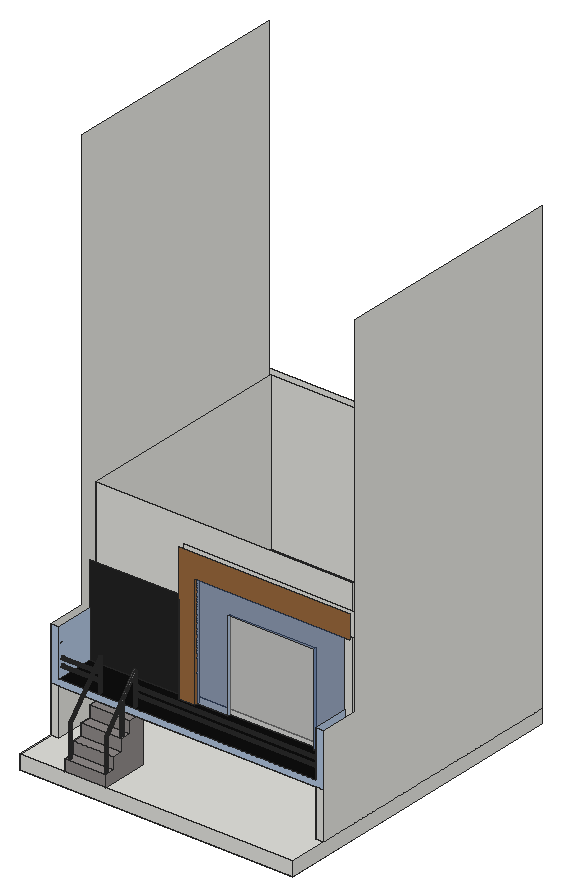
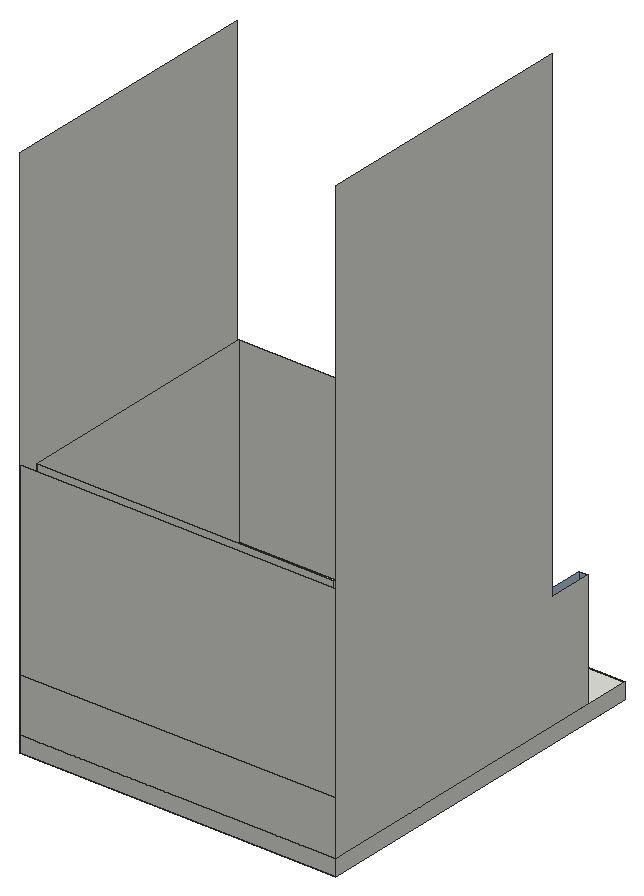
# SketchUp Ruby script. Lengths in inches.
U = 1.inch
M = Sketchup.active_model
def pt(a) = Geom::Point3d.new(a.map { |v| v * U })
def face(e, loops, mat)
  f = e.add_face(loops[0].map { |a| pt(a) })
  loops[1..].each { |l| e.add_face(l.map { |a| pt(a) }).erase! }
  f.material = f.back_material = mat if mat
  f
end
# faces: each face lists its corners as indices into pts; further lists are holes
def faces(e, pts, list, mat = nil) = list.each { |f| face(e, (f[0].is_a?(Array) ? f : [f]).map { |l| l.map { |i| pts[i] } }, mat) }
# xy, xz, yz: faces in a plane at the given z, y or x. An outline is a flat list of corners, or four numbers for a rectangle; further outlines are holes
def ring(l) = l.size == 4 ? [[l[0], l[1]], [l[2], l[1]], [l[2], l[3]], [l[0], l[3]]] : l.each_slice(2).to_a
def flat(e, list, mat, &to3) = list.each { |f| face(e, (f[0].is_a?(Array) ? f : [f]).map { |l| ring(l).map { |u, v| to3.(u, v) } }, mat) }
def xy(e, z, list, mat = nil) = flat(e, list, mat) { |x, y| [x, y, z] }
def xz(e, y, list, mat = nil) = flat(e, list, mat) { |x, z| [x, y, z] }
def yz(e, x, list, mat = nil) = flat(e, list, mat) { |y, z| [x, y, z] }
def lines(e, pts, list) = list.each { |a, b| e.add_line(pt(pts[a]), pt(pts[b])) }
# prism: a flat outline (further loops are holes) pulled along v
def prism(e, loops, v, mat = nil)
  f = face(e, loops, mat); d = Geom::Vector3d.new(v.map { |x| x * U })
  f.pushpull(f.normal.samedirection?(d) ? d.length : -d.length)
end
def box(e, o, s, mat = nil) = prism(e, [[o, [o[0] + s[0], o[1], o[2]], [o[0] + s[0], o[1] + s[1], o[2]], [o[0], o[1] + s[1], o[2]]]], [0, 0, s[2]], mat)
def at(x, y, z, deg = 0) = Geom::Transformation.translation(pt([x, y, z])) * Geom::Transformation.rotation(ORIGIN, Z_AXIS, deg.degrees)
def axes(o, x, y, z) = Geom::Transformation.new([*x, 0, *y, 0, *z, 0, *pt(o).to_a, 1])
def part(name) = M.definitions.add(name)
# library, detail: a bought-in or finely detailed component or shape, given as its bounding box
def library(name, o, s) = part(name).tap { |d| box(d.entities, o, s) }
def detail(e, o, s) = box(e.add_group.entities, o, s)
def put(e, d, t, mat = nil) = e.add_instance(d, t).tap { |i| i.material = mat if mat }
def group(e, t, mat = nil) = e.add_group.tap { |g| g.transformation = t; g.material = mat if mat }.entities
root = M.entities
M.materials.add("[0099_LightSteelBlue]").color = [176, 196, 222]
M.materials.add("[0136_Charcoal]").color = [35, 35, 35]
M.materials.add("[Granite Dark Gray]").color = [15, 15, 15]
M.materials.add("[Metal Corrugated Shiny]").color = [124, 124, 124]
M.materials.add("[Stone Marble]").color = [143, 138, 136]
M.materials.add("[Translucent Glass Blue]").color = [59, 88, 140]
M.materials["[Translucent Glass Blue]"].alpha = 0.5
M.materials.add("[Translucent Glass Gray]").color = [173, 173, 173]
M.materials["[Translucent Glass Gray]"].alpha = 0.5
M.materials.add("[Wood Floor]").color = [155, 105, 61]
xy(root,0,[[0,0,420,480]])
xy(root,21,[[0,0,69.34,0,69.34,72,132,72,132,0,420,0,420,60,408,60,408,468,12,468,12,60,0,60],[0,60,0,480,420,480,420,60,408,60,408,468,12,468,12,60]])
xy(root,39,[[73.02,4.13,72.5,4.2,72.02,4.4,71.61,4.71,71.29,5.13,71.09,5.61,71.02,6.13,71.09,6.64,71.29,7.13,71.61,7.54,72.02,7.86,72.5,8.06,73.02,8.13,73.54,8.06,74.02,7.86,74.44,7.54,74.75,7.13,74.95,6.64,75.02,6.13,74.95,5.61,74.75,5.13,74.44,4.71,74.02,4.4,73.54,4.2],[128.75,4.13,128.77,4.13,129,4.16],[128.49,4.16,128.23,4.21,128.25,4.2],[129.26,4.19,129.29,4.2,129.51,4.29],[127.99,4.3,127.75,4.41,127.77,4.4],
  [129.75,4.39,129.77,4.4,129.96,4.54],[127.54,4.57,127.34,4.73,127.36,4.71],[130.17,4.7,130.19,4.71,130.33,4.9],[127.18,4.94,127.03,5.15,127.04,5.13],[130.49,5.11,130.5,5.13,130.59,5.35],
  [126.93,5.39,126.84,5.64,126.84,5.61],[130.69,5.59,130.7,5.61,130.73,5.84],[126.8,5.89,126.77,6.15,126.77,6.13],[130.77,6.1,130.77,6.13,130.74,6.36],[126.81,6.41,126.85,6.67,126.84,6.64],
  [130.71,6.62,130.7,6.64,130.61,6.86],[126.95,6.91,127.05,7.15,127.04,7.13],[130.51,7.1,130.5,7.13,130.36,7.3125],[127.21,7.35,127.38,7.56,127.36,7.54],[130.2,7.52,130.19,7.54,130,7.68],
  [127.58,7.72,127.79,7.87,127.77,7.86],[129.79,7.84,129.77,7.86,129.55,7.95],[128.04,7.97,128.28,8.0625,128.25,8.06],[129.3125,8.05,129.29,8.06,129.06,8.09],[128.54,8.1,128.8,8.125,128.77,8.13]])
xy(root,39,[[[69.34,0,132,16],[128.72,4.13,128.49,4.16,128.25,4.2,128.23,4.21,128.2,4.21,127.99,4.3,127.77,4.4,127.73,4.42,127.54,4.57,127.36,4.71,127.32,4.75,127.04,5.13,127.03,5.15,127.01,5.17,126.93,5.39,126.84,5.61,126.84,5.64,126.83,5.66,126.8,5.89,126.77,6.13,126.77,6.18,126.81,6.41,126.84,6.64,126.85,6.67,126.85,6.69,126.95,6.91,127.04,7.13,127.05,7.15,127.07,7.17,127.21,7.35,127.36,7.54,127.38,7.56,127.39,7.58,127.77,7.86,127.79,7.87,127.82,7.88,128.04,7.97,128.25,8.06,128.28,8.0625,128.3,8.07,128.54,8.1,128.77,8.13,128.8,8.125,128.82,8.125,129.06,8.09,129.29,8.06,129.3125,8.05,129.34,8.05,129.55,7.95,129.77,7.86,129.79,7.84,129.82,7.83,130,7.68,130.19,7.54,130.2,7.52,130.22,7.5,130.36,7.3125,130.5,7.13,130.51,7.1,130.53,7.08,130.61,6.86,130.7,6.64,130.72,6.6,130.74,6.36,130.77,6.13,130.77,6.08,130.73,5.84,130.7,5.61,130.69,5.59,130.6875,5.56,130.59,5.35,130.5,5.13,130.49,5.11,130.48,5.08,130.33,4.9,130.19,4.71,130.17,4.7,130.15,4.68,129.77,4.4,129.75,4.39,129.73,4.37,129.51,4.29,129.29,4.2,129.26,4.19,129.24,4.18,129,4.16,128.77,4.13],[73.02,4.13,72.5,4.2,72.02,4.4,71.61,4.71,71.29,5.13,71.09,5.61,71.02,6.13,71.09,6.64,71.29,7.13,71.61,7.54,72.02,7.86,72.5,8.06,73.02,8.13,73.54,8.06,74.02,7.86,74.44,7.54,74.75,7.13,74.95,6.64,75.02,6.13,74.95,5.61,74.75,5.13,74.44,4.71,74.02,4.4,73.54,4.2]]],"[Stone Marble]")
xy(root,57,[[69.34,16,132,30.4375]],"[Stone Marble]")
xy(root,75,[[127.2,35.08,126.68,35.15,126.2,35.35,125.78,35.67,125.46,36.08,125.26,36.5625,125.2,37.08,125.26,37.6,125.46,38.08,125.78,38.49,126.2,38.8125,126.68,39.01,127.2,39.08,127.71,39.01,128.2,38.8125,128.61,38.49,128.93,38.08,129.13,37.6,129.2,37.08,129.13,36.5625,128.93,36.08,128.61,35.67,128.2,35.35,127.71,35.15]])
xy(root,75,[[[69.34,30.4375,132,47.125],[127.2,35.08,126.68,35.15,126.2,35.35,125.78,35.67,125.46,36.08,125.26,36.5625,125.2,37.08,125.26,37.6,125.46,38.08,125.78,38.49,126.2,38.8125,126.68,39.01,127.2,39.08,127.71,39.01,128.2,38.8125,128.61,38.49,128.93,38.08,129.13,37.6,129.2,37.08,129.13,36.5625,128.93,36.08,128.61,35.67,128.2,35.35,127.71,35.15]]],"[Stone Marble]")
xy(root,93,[[12,60,12,468,408,468,408,60,132,60,132,72,69.34,72,69.34,60],[69.34,60,132,72]])
xy(root,93,[[69.34,47.125,132,60]],"[Stone Marble]")
xy(root,103,[[72.44,62.83,71.92,62.9,71.44,63.1,71.03,63.42,70.71,63.83,70.51,64.32,70.44,64.83,70.51,65.35,70.71,65.83,71.03,66.25,71.44,66.57,71.92,66.77,72.44,66.83,72.96,66.77,73.44,66.57,73.86,66.25,74.17,65.83,74.375,65.35,74.44,64.83,74.375,64.32,74.17,63.83,73.86,63.42,73.44,63.1,72.96,62.9],[126.03,62.85,125.51,62.86,125.01,63.01,124.56,63.28,124.2,63.66,123.95,64.11,123.83,64.62,123.84,65.14,123.99,65.64,124.26,66.09,124.64,66.45,125.1,66.7,125.6,66.82,126.125,66.81,126.625,66.66,127.07,66.39,127.43,66.01,127.68,65.55,127.8,65.05,127.79,64.52,127.64,64.02,127.37,63.58,126.99,63.22,126.54,62.97],[156,111,180,120],[12,132,408,468]])
xy(root,103,[[[12,60,408,60,408,116,360,116,360,120,228,120,228,116,180,116,180,111,156,111,156,120,12,120],[72.44,62.83,71.92,62.9,71.44,63.1,71.03,63.42,70.71,63.83,70.51,64.32,70.44,64.83,70.51,65.35,70.71,65.83,71.03,66.25,71.44,66.57,71.92,66.77,72.44,66.83,72.96,66.77,73.44,66.57,73.86,66.25,74.17,65.83,74.375,65.35,74.44,64.83,74.375,64.32,74.17,63.83,73.86,63.42,73.44,63.1,72.96,62.9],[126.03,62.85,125.51,62.86,125.01,63.01,124.56,63.28,124.2,63.66,123.95,64.11,123.83,64.62,123.84,65.14,123.99,65.64,124.26,66.09,124.64,66.45,125.1,66.7,125.6,66.82,126.125,66.81,126.625,66.66,127.07,66.39,127.43,66.01,127.68,65.55,127.8,65.05,127.79,64.52,127.64,64.02,127.37,63.58,126.99,63.22,126.54,62.97]]],"[Granite Dark Gray]")
xy(root,121.24,[[127.2,35.08,127.71,35.15,128.2,35.35,128.61,35.67,128.93,36.08,129.13,36.5625,129.2,37.08,129.13,37.6,128.93,38.08,128.61,38.49,128.2,38.8125,127.71,39.01,127.2,39.08,126.68,39.01,126.2,38.8125,125.78,38.49,125.46,38.08,125.26,37.6,125.2,37.08,125.26,36.5625,125.46,36.08,125.78,35.67,126.2,35.35,126.68,35.15]])
xz(root,0,[[0,0,420,21]])
xz(root,0,[[69.34,21,132,39]],"[Stone Marble]")
xz(root,16,[[69.34,39,132,57]],"[Stone Marble]")
xz(root,30.4375,[[69.34,57,132,75]],"[Stone Marble]")
xz(root,47.125,[[69.34,75,132,93]],"[Stone Marble]")
xz(root,60,[[0,21,12,93],[408,21,420,93]])
xz(root,60,[[0,93,420,93,420,175,408,175,408,103,12,103,12,175,0,175]],"[0099_LightSteelBlue]")
xz(root,72,[[69.34,21,132,93]])
xz(root,111,[[156,103,180,103,180,277,420,277,420,313,156,313]],"[Wood Floor]")
xz(root,116,[[180,103,228,103,228,241,360,241,360,103,408,103,408,277,180,277]],"[Translucent Glass Blue]")
xz(root,120,[[156,103,156,313,420,313,420,277,180,277,180,103]])
xz(root,120,[[12,103,156,241]],"[0136_Charcoal]")
xz(root,120,[[228,103,360,241]],"[Translucent Glass Gray]")
xz(root,132,[[12,103,408,343]])
xz(root,468,[[12,21,408,93],[12,103,408,343]])
xz(root,480,[[0,0,420,21],[0,21,420,93],[0,93,420,343]])
yz(root,0,[[0,0,480,21],[60,21,60,175,120,175,120,823,480,823,480,21]])
yz(root,12,[[60,21,468,93],[132,103,468,343],[64.83,116.9375,64.32,117.01,63.83,117.21,63.42,117.52,63.1,117.9375,62.9,118.42,62.83,118.9375,62.9,119.46,63.1,119.9375,63.42,120.35,63.83,120.67,64.32,120.87,64.83,120.9375,65.35,120.87,65.83,120.67,66.25,120.35,66.57,119.9375,66.77,119.46,66.83,118.9375,66.77,118.42,66.57,117.9375,66.25,117.52,65.83,117.21,65.35,117.01],[64.83,127.875,64.32,127.94,63.83,128.14,63.42,128.46,63.1,128.875,62.9,129.36,62.83,129.875,62.9,130.39,63.1,130.875,63.42,131.29,63.83,131.61,64.32,131.81,64.83,131.875,65.35,131.81,65.83,131.61,66.25,131.29,66.57,130.875,66.77,130.39,66.83,129.875,66.77,129.36,66.57,128.875,66.25,128.46,65.83,128.14,65.35,127.94]])
yz(root,12,[[[60,103,120,175],[64.83,116.9375,64.32,117.01,63.83,117.21,63.42,117.52,63.1,117.9375,62.9,118.42,62.83,118.9375,62.9,119.46,63.1,119.9375,63.42,120.35,63.83,120.67,64.32,120.87,64.83,120.9375,65.35,120.87,65.83,120.67,66.25,120.35,66.57,119.9375,66.77,119.46,66.83,118.9375,66.77,118.42,66.57,117.9375,66.25,117.52,65.83,117.21,65.35,117.01],[64.83,127.875,64.32,127.94,63.83,128.14,63.42,128.46,63.1,128.875,62.9,129.36,62.83,129.875,62.9,130.39,63.1,130.875,63.42,131.29,63.83,131.61,64.32,131.81,64.83,131.875,65.35,131.81,65.83,131.61,66.25,131.29,66.57,130.875,66.77,130.39,66.83,129.875,66.77,129.36,66.57,128.875,66.25,128.46,65.83,128.14,65.35,127.94],[64.83,138.5625,64.32,138.63,63.83,138.83,63.42,139.15,63.1,139.5625,62.9,140.05,62.83,140.5625,62.9,141.08,63.1,141.5625,63.42,141.98,63.83,142.3,64.32,142.5,64.83,142.5625,65.35,142.5,65.83,142.3,66.25,141.98,66.57,141.5625,66.77,141.08,66.83,140.5625,66.77,140.05,66.57,139.5625,66.25,139.15,65.83,138.83,65.35,138.63],[64.83,149.25,64.32,149.32,63.83,149.52,63.42,149.84,63.1,150.25,62.9,150.73,62.83,151.25,62.9,151.77,63.1,152.25,63.42,152.67,63.83,152.98,64.32,153.18,64.83,153.25,65.35,153.18,65.83,152.98,66.25,152.67,66.57,152.25,66.77,151.77,66.83,151.25,66.77,150.73,66.57,150.25,66.25,149.84,65.83,149.52,65.35,149.32]]],"[0099_LightSteelBlue]")
yz(root,69.34,[[0,21,0,39,16,39,16,57,30.4375,57,30.4375,75,47.125,75,47.125,93,72,93,72,21]],"[Stone Marble]")
yz(root,132,[[0,21,72,21,72,93,47.125,93,47.125,75,30.4375,75,30.4375,57,16,57,16,39,0,39]],"[Stone Marble]")
yz(root,156,[[111,103,120,241]])
yz(root,180,[[116,103,120,277]])
yz(root,180,[[111,103,116,277]],"[Wood Floor]")
yz(root,228,[[116,103,120,241]],"[0099_LightSteelBlue]")
yz(root,360,[[116,103,120,241]],"[0099_LightSteelBlue]")
yz(root,408,[[60,21,468,93],[132,103,468,343],[64.83,117.19,65.29,117.25,65.71,117.42,66.07,117.7,66.35,118.06,66.52,118.49,66.58,118.9375,66.52,119.39,66.35,119.8125,66.07,120.18,65.71,120.45,65.29,120.63,64.83,120.6875,64.38,120.63,63.96,120.45,63.6,120.18,63.32,119.8125,63.14,119.39,63.08,118.9375,63.14,118.49,63.32,118.06,63.6,117.7,63.96,117.42,64.38,117.25],[64.83,127.98,65.32,128.05,65.78,128.24,66.17,128.54,66.47,128.93,66.66,129.39,66.73,129.875,66.66,130.37,66.47,130.82,66.17,131.21,65.78,131.52,65.32,131.7,64.83,131.77,64.34,131.7,63.89,131.52,63.5,131.21,63.2,130.82,63.01,130.37,62.94,129.875,63.01,129.39,63.2,128.93,63.5,128.54,63.89,128.24,64.34,128.05]])
yz(root,408,[[[60,103,116,175],[64.83,138.5625,65.35,138.63,65.83,138.83,66.25,139.15,66.57,139.5625,66.77,140.05,66.83,140.5625,66.77,141.08,66.57,141.5625,66.25,141.98,65.83,142.3,65.35,142.5,64.83,142.5625,64.32,142.5,63.83,142.3,63.42,141.98,63.1,141.5625,62.9,141.08,62.83,140.5625,62.9,140.05,63.1,139.5625,63.42,139.15,63.83,138.83,64.32,138.63],[64.83,149.25,65.35,149.32,65.83,149.52,66.25,149.84,66.57,150.25,66.77,150.73,66.83,151.25,66.77,151.77,66.57,152.25,66.25,152.67,65.83,152.98,65.35,153.18,64.83,153.25,64.32,153.18,63.83,152.98,63.42,152.67,63.1,152.25,62.9,151.77,62.83,151.25,62.9,150.73,63.1,150.25,63.42,149.84,63.83,149.52,64.32,149.32],[64.83,127.98,65.32,128.05,65.78,128.24,66.17,128.54,66.47,128.93,66.66,129.39,66.73,129.875,66.66,130.37,66.47,130.82,66.17,131.21,65.78,131.52,65.32,131.7,64.83,131.77,64.34,131.7,63.89,131.52,63.5,131.21,63.2,130.82,63.01,130.37,62.94,129.875,63.01,129.39,63.2,128.93,63.5,128.54,63.89,128.24,64.34,128.05],[64.83,117.19,65.29,117.25,65.71,117.42,66.07,117.7,66.35,118.06,66.52,118.49,66.58,118.9375,66.52,119.39,66.35,119.8125,66.07,120.18,65.71,120.45,65.29,120.63,64.83,120.6875,64.38,120.63,63.96,120.45,63.6,120.18,63.32,119.8125,63.14,119.39,63.08,118.9375,63.14,118.49,63.32,118.06,63.6,117.7,63.96,117.42,64.38,117.25]]],"[0099_LightSteelBlue]")
yz(root,420,[[0,0,480,21],[60,21,480,21,480,715,120,715,120,175,60,175]])
p = [[72.5,4.2,39],[73.02,4.13,39],[73.02,4.13,87.78],[72.5,4.2,87.75],[73.54,4.2,39],[73.54,4.2,87.75],
  [128.72,4.13,87.77],[128.2,4.21,87.73],[128.2,4.21,39],[128.23,4.21,39],[128.49,4.16,39],[128.72,4.13,39],
  [129.24,4.18,87.76],[128.75,4.13,39],[129,4.16,39],[129.24,4.18,39],[72.02,4.4,39],[72.02,4.4,87.67],
  [74.02,4.4,39],[74.02,4.4,87.68],[127.73,4.42,87.64],[127.73,4.42,39],[127.75,4.41,39],[127.99,4.3,39],
  [129.73,4.37,87.69],[129.26,4.19,39],[129.51,4.29,39],[129.73,4.37,39],[71.61,4.71,39],[71.61,4.71,87.54],
  [74.44,4.71,39],[74.44,4.71,87.55],[127.32,4.75,87.5],[127.32,4.75,39],[127.34,4.73,39],[127.54,4.57,39],
  [130.15,4.68,87.58],[129.75,4.39,39],[129.96,4.54,39],[130.15,4.68,39],[71.29,5.13,39],[71.29,5.13,87.38],
  [74.75,5.13,39],[74.75,5.13,87.39],[127.01,5.17,87.33],[127.01,5.17,39],[127.03,5.15,39],[127.18,4.94,39],
  [130.48,5.08,87.44],[130.17,4.7,39],[130.33,4.9,39],[130.48,5.08,39],[71.09,5.61,39],[71.09,5.61,87.19],
  [74.95,5.61,39],[74.95,5.61,87.21],[130.6875,5.56,87.26],[130.49,5.11,39],[130.59,5.35,39],[130.6875,5.56,39],
  [126.83,5.66,87.14],[126.83,5.66,39],[126.84,5.64,39],[126.93,5.39,39],[71.02,6.13,39],[71.02,6.13,86.99],
  [75.02,6.13,39],[75.02,6.13,87.01],[130.77,6.08,87.06],[130.69,5.59,39],[130.73,5.84,39],[130.77,6.08,39],
  [126.77,6.18,86.94],[126.77,6.18,39],[126.77,6.15,39],[126.8,5.89,39],[71.09,6.64,39],[71.09,6.64,86.79],
  [74.95,6.64,39],[74.95,6.64,86.81],[130.72,6.6,86.86],[130.77,6.1,39],[130.74,6.36,39],[130.72,6.6,39],
  [126.85,6.69,86.74],[126.85,6.69,39],[126.85,6.67,39],[126.81,6.41,39],[71.29,7.13,39],[71.29,7.13,86.61],
  [74.75,7.13,39],[74.75,7.13,86.62],[130.53,7.08,86.67],[130.71,6.62,39],[130.61,6.86,39],[130.53,7.08,39],
  [127.07,7.17,86.56],[127.07,7.17,39],[127.05,7.15,39],[126.95,6.91,39],[71.61,7.54,39],[71.61,7.54,86.45],
  [74.44,7.54,39],[74.44,7.54,86.46],[130.22,7.5,86.5],[130.51,7.1,39],[130.36,7.3125,39],[130.22,7.5,39],
  [127.39,7.58,86.42],[127.39,7.58,39],[127.38,7.56,39],[127.21,7.35,39],[72.02,7.86,39],[72.02,7.86,86.32],
  [74.02,7.86,39],[74.02,7.86,86.33],[129.82,7.83,86.36],[130.2,7.52,39],[130,7.68,39],[129.82,7.83,39],
  [127.82,7.88,86.31],[127.82,7.88,39],[127.79,7.87,39],[127.58,7.72,39],[129.34,8.05,86.27],[129.79,7.84,39],
  [129.55,7.95,39],[129.34,8.05,39],[72.5,8.06,39],[72.5,8.06,86.25],[73.54,8.06,39],[73.54,8.06,86.25],
  [128.3,8.07,86.24],[128.3,8.07,39],[128.28,8.0625,39],[128.04,7.97,39],[128.82,8.125,86.23],[129.3125,8.05,39],
  [129.06,8.09,39],[128.82,8.125,39],[73.02,8.13,39],[73.02,8.13,86.22],[128.8,8.125,39],[128.54,8.1,39],
  [126.2,35.35,75],[126.68,35.15,75],[126.68,35.15,121.24],[126.2,35.35,121.24],[127.2,35.08,75],[127.2,35.08,121.24],
  [127.71,35.15,75],[127.71,35.15,121.24],[128.2,35.35,75],[128.2,35.35,121.24],[125.78,35.67,75],[125.78,35.67,121.24],
  [128.61,35.67,75],[128.61,35.67,121.24],[125.46,36.08,75],[125.46,36.08,121.24],[128.93,36.08,75],[128.93,36.08,121.24],
  [125.26,36.5625,75],[125.26,36.5625,121.24],[129.13,36.5625,75],[129.13,36.5625,121.24],[125.2,37.08,75],[125.2,37.08,121.24],
  [129.2,37.08,75],[129.2,37.08,121.24],[125.26,37.6,75],[125.26,37.6,121.24],[129.13,37.6,75],[129.13,37.6,121.24],
  [125.46,38.08,75],[125.46,38.08,121.24],[128.93,38.08,75],[128.93,38.08,121.24],[125.78,38.49,75],[125.78,38.49,121.24],
  [128.61,38.49,75],[128.61,38.49,121.24],[126.2,38.8125,75],[126.2,38.8125,121.24],[128.2,38.8125,75],[128.2,38.8125,121.24],
  [126.68,39.01,75],[126.68,39.01,121.24],[127.71,39.01,75],[127.71,39.01,121.24],[127.2,39.08,75],[127.2,39.08,121.24],
  [71.45,66.11,150.08],[71.93,66.26,149.95],[126.26,38.37,120.02],[126.75,38.51,119.91],[127.27,38.56,119.89],[127.79,38.5,119.97],
  [72.45,66.31,149.9],[72.96,66.26,149.95],[71.03,65.875,150.29],[73.45,66.12,150.09],[73.86,65.88,150.31],[125.84,38.13,120.22],
  [128.26,38.35,120.125],[70.71,65.57,150.57],[125.51,37.83,120.48],[128.66,38.12,120.36],[74.18,65.58,150.59],[128.96,37.81,120.66],
  [70.51,65.21,150.89],[74.375,65.22,150.92],[125.29,37.47,120.79],[125.2,37.09,121.14],[129.15,37.45,120.99],[70.44,64.83,151.24],
  [70.44,64.83,151.23],[74.44,64.84,151.27],[74.44,64.83,151.26],[125.25,36.71,121.49],[129.19,37.07,121.34],[70.51,64.32,151.45],
  [70.51,64.45,151.59],[74.44,64.83,151.27],[74.37,64.46,151.61],[74.375,64.32,151.46],[125.43,36.35,121.83],[129.11,36.6875,121.6875],
  [70.71,63.83,151.63],[70.71,64.09,151.91],[74.17,64.1,151.9375],[74.17,63.83,151.65],[125.73,36.04,122.12],[128.89,36.33,122],
  [71.03,63.42,151.8],[71.02,63.79,152.2],[73.85,63.79,152.22],[73.86,63.42,151.81],[128.55,36.03,122.27],[71.44,63.1,151.92],
  [71.4375,63.55,152.41],[126.13,35.81,122.36],[126.6,35.66,122.52],[73.4375,63.56,152.43],[73.44,63.1,151.93],[128.13,35.8,122.46],
  [72.44,62.83,152.03],[72.4375,63.36,152.6],[71.92,63.41,152.55],[71.92,62.9,152],[127.12,35.6,122.59],[72.95,63.41,152.56],
  [72.96,62.9,152],[127.64,35.65,122.57],[71.92,62.9,103],[72.44,62.83,103],[72.44,62.83,118.9375],[72.44,62.83,129.875],
  [72.44,62.83,140.5625],[72.44,62.83,153],[71.92,62.9,153],[71.92,62.9,141.08],[71.92,62.9,140.05],[71.92,62.9,130.39],
  [71.92,62.9,129.36],[71.92,62.9,119.46],[71.92,62.9,118.42],[72.96,62.9,103],[72.96,62.9,153],[125.51,62.86,103],
  [126.03,62.85,103],[126.03,62.85,151.31],[125.51,62.86,151.31],[126.54,62.97,103],[126.54,62.97,151.31],[71.44,63.1,103],
  [71.44,63.1,153],[71.44,63.1,141.5625],[71.44,63.1,139.5625],[71.44,63.1,130.875],[71.44,63.1,128.875],[71.44,63.1,119.9375],
  [71.44,63.1,117.9375],[73.44,63.1,103],[73.44,63.1,153],[125.01,63.01,103],[125.01,63.01,151.31],[124.56,63.28,103],
  [124.56,63.28,151.31],[126.99,63.22,103],[126.99,63.22,151.31],[71.03,63.42,103],[71.03,63.42,153],[71.03,63.42,141.98],
  [71.03,63.42,139.15],[71.03,63.42,131.29],[71.03,63.42,128.46],[71.03,63.42,120.35],[71.03,63.42,117.52],[73.86,63.42,103],
  [73.86,63.42,153],[127.37,63.58,103],[127.37,63.58,151.31],[124.2,63.66,103],[124.2,63.66,151.31],[70.71,63.83,103],
  [70.71,63.83,153],[70.71,63.83,152.98],[70.71,63.83,149.52],[70.71,63.83,142.3],[70.71,63.83,138.83],[70.71,63.83,131.61],
  [70.71,63.83,128.14],[70.71,63.83,120.67],[70.71,63.83,117.21],[74.17,63.83,103],[74.17,63.83,153],[127.64,64.02,103],
  [127.64,64.02,151.31],[123.95,64.11,103],[123.95,64.11,151.31],[70.51,64.32,103],[70.51,64.32,153],[70.51,64.32,149.32],
  [70.51,64.32,142.5],[70.51,64.32,138.63],[70.51,64.32,131.81],[70.51,64.32,127.94],[70.51,64.32,120.87],[70.51,64.32,117.01],
  [74.375,64.32,103],[74.375,64.32,153],[127.79,64.52,103],[127.79,64.52,151.31],[123.83,64.62,103],[123.83,64.62,151.31],
  [70.44,64.83,103],[70.44,64.83,153],[70.44,64.83,151.25],[70.44,64.83,149.25],[70.44,64.83,142.5625],[70.44,64.83,140.5625],
  [70.44,64.83,138.5625],[70.44,64.83,131.875],[70.44,64.83,129.875],[70.44,64.83,127.875],[70.44,64.83,120.9375],[70.44,64.83,118.9375],
  [70.44,64.83,116.9375],[74.44,64.83,103],[74.44,64.83,153],[127.8,65.05,103],[127.8,65.05,151.31],[127.8,64.83,151.31],
  [123.84,65.14,103],[123.84,65.14,151.31],[70.51,65.35,103],[70.51,65.35,153],[70.51,65.35,149.32],[70.51,65.35,142.5],
  [70.51,65.35,138.63],[70.51,65.35,131.81],[70.51,65.35,127.94],[70.51,65.35,120.87],[70.51,65.35,117.01],[74.375,65.35,103],
  [74.375,65.35,153],[127.68,65.55,103],[127.68,65.55,151.31],[123.99,65.64,103],[123.99,65.64,151.31],[70.71,65.83,103],
  [70.71,65.83,153],[70.71,65.83,152.98],[70.71,65.83,149.52],[70.71,65.83,142.3],[70.71,65.83,138.83],[70.71,65.83,131.61],
  [70.71,65.83,128.14],[70.71,65.83,120.67],[70.71,65.83,117.21],[74.17,65.83,103],[74.17,65.83,153],[124.26,66.09,103],
  [124.26,66.09,151.31],[127.43,66.01,103],[127.43,66.01,151.31],[71.03,66.25,103],[71.03,66.25,153],[71.03,66.25,141.98],
  [71.03,66.25,139.15],[71.03,66.25,131.29],[71.03,66.25,128.46],[71.03,66.25,120.35],[71.03,66.25,117.52],[73.86,66.25,103],
  [73.86,66.25,153],[127.07,66.39,103],[127.07,66.39,151.31],[124.64,66.45,103],[124.64,66.45,151.31],[71.44,66.57,103],
  [71.44,66.57,153],[71.44,66.57,141.5625],[71.44,66.57,139.5625],[71.44,66.57,130.875],[71.44,66.57,128.875],[71.44,66.57,119.9375],
  [71.44,66.57,117.9375],[73.44,66.57,103],[73.44,66.57,153],[125.1,66.7,103],[125.1,66.7,151.31],[126.625,66.66,103],
  [126.625,66.66,151.31],[71.92,66.77,103],[71.92,66.77,153],[71.92,66.77,141.08],[71.92,66.77,140.05],[71.92,66.77,130.39],
  [71.92,66.77,129.36],[71.92,66.77,119.46],[71.92,66.77,118.42],[72.96,66.77,103],[72.96,66.77,153],[125.6,66.82,103],
  [125.6,66.82,151.31],[126.125,66.81,103],[126.125,66.81,151.31],[72.44,66.83,103],[72.44,66.83,153],[72.44,66.83,140.5625],
  [72.44,66.83,129.875],[72.44,66.83,118.9375],[12,64.32,117.01],[12,64.83,116.9375],[72.44,64.83,116.9375],[72.44,64.32,117.01],
  [12,65.35,117.01],[72.44,65.35,117.01],[12,63.83,117.21],[72.44,63.83,117.21],[12,65.83,117.21],[72.44,65.83,117.21],
  [12,63.42,117.52],[72.44,63.42,117.52],[408,64.38,117.25],[408,63.96,117.42],[125.82,63.96,117.42],[125.82,64.38,117.25],
  [408,64.83,117.19],[125.82,64.83,117.19],[127.8,64.83,117.19],[408,65.29,117.25],[125.82,65.29,117.25],[408,65.71,117.42],
  [125.82,65.71,117.42],[12,66.25,117.52],[72.44,66.25,117.52],[408,63.6,117.7],[125.82,63.6,117.7],[408,66.07,117.7],
  [125.82,66.07,117.7],[12,63.1,117.9375],[72.44,63.1,117.9375],[12,66.57,117.9375],[72.44,66.57,117.9375],[408,63.32,118.06],
  [125.82,63.32,118.06],[408,66.35,118.06],[125.82,66.35,118.06],[12,62.9,118.42],[72.44,62.9,118.42],[12,66.77,118.42],
  [72.44,66.77,118.42],[408,63.14,118.49],[125.82,63.14,118.49],[408,66.52,118.49],[125.82,66.52,118.49],[12,62.83,118.9375],
  [12,66.83,118.9375],[408,63.08,118.9375],[125.82,63.08,118.9375],[408,66.58,118.9375],[125.82,66.58,118.9375],[12,62.9,119.46],
  [72.44,62.9,119.46],[408,63.14,119.39],[125.82,63.14,119.39],[408,66.52,119.39],[125.82,66.52,119.39],[12,66.77,119.46],
  [72.44,66.77,119.46],[408,63.32,119.8125],[125.82,63.32,119.8125],[408,66.35,119.8125],[125.82,66.35,119.8125],[12,63.1,119.9375],
  [72.44,63.1,119.9375],[12,66.57,119.9375],[72.44,66.57,119.9375],[408,63.6,120.18],[125.82,63.6,120.18],[408,66.07,120.18],
  [125.82,66.07,120.18],[124.85,66.77,150.73],[125.36,66.57,150.25],[125.9,66.25,149.84],[126.43,65.83,149.52],[12,63.42,120.35],
  [72.44,63.42,120.35],[12,66.25,120.35],[72.44,66.25,120.35],[124.41,66.83,151.25],[126.92,65.35,149.32],[127.33,64.83,149.25],
  [124.07,66.77,151.77],[408,63.96,120.45],[125.82,63.96,120.45],[408,65.71,120.45],[125.82,65.71,120.45],[127.65,64.32,149.32],
  [12,63.83,120.67],[72.44,63.83,120.67],[12,65.83,120.67],[72.44,65.83,120.67],[123.84,66.57,152.25],[408,64.38,120.63],
  [125.82,64.38,120.63],[408,65.29,120.63],[125.82,65.29,120.63],[408,64.83,120.6875],[127.8,64.83,120.6875],[125.82,64.83,120.6875],
  [127.83,63.83,149.52],[12,64.32,120.87],[72.44,64.32,120.87],[12,65.35,120.87],[72.44,65.35,120.87],[123.75,66.25,152.67],
  [12,64.83,120.9375],[72.44,64.83,120.9375],[127.88,63.42,149.84],[123.8,65.83,152.98],[127.79,63.1,150.25],[123.99,65.35,153.18],
  [127.57,62.9,150.73],[124.3,64.83,153.25],[127.22,62.83,151.25],[124.71,64.32,153.18],[126.78,62.9,151.77],[125.2,63.83,152.98],
  [125.74,63.42,152.67],[126.27,63.1,152.25],[12,63.83,128.14],[12,64.32,127.94],[72.44,64.32,127.94],[72.44,63.83,128.14],
  [12,64.83,127.875],[72.44,64.83,127.875],[12,65.35,127.94],[72.44,65.35,127.94],[12,65.83,128.14],[72.44,65.83,128.14],
  [408,64.34,128.05],[408,63.89,128.24],[125.82,63.89,128.24],[125.82,64.34,128.05],[408,64.83,127.98],[125.82,64.83,127.98],
  [127.8,64.83,127.98],[408,65.32,128.05],[125.82,65.32,128.05],[408,65.78,128.24],[125.82,65.78,128.24],[12,63.42,128.46],
  [72.44,63.42,128.46],[12,66.25,128.46],[72.44,66.25,128.46],[408,63.5,128.54],[125.82,63.5,128.54],[408,66.17,128.54],
  [125.82,66.17,128.54],[12,63.1,128.875],[72.44,63.1,128.875],[408,63.2,128.93],[125.82,63.2,128.93],[12,66.57,128.875],
  [72.44,66.57,128.875],[408,66.47,128.93],[125.82,66.47,128.93],[12,62.9,129.36],[72.44,62.9,129.36],[408,63.01,129.39],
  [125.82,63.01,129.39],[408,66.66,129.39],[125.82,66.66,129.39],[12,66.77,129.36],[72.44,66.77,129.36],[12,62.83,129.875],
  [408,62.94,129.875],[125.82,62.94,129.875],[408,66.73,129.875],[125.82,66.73,129.875],[12,66.83,129.875],[12,62.9,130.39],
  [72.44,62.9,130.39],[408,63.01,130.37],[125.82,63.01,130.37],[408,66.66,130.37],[125.82,66.66,130.37],[12,66.77,130.39],
  [72.44,66.77,130.39],[12,63.1,130.875],[72.44,63.1,130.875],[408,63.2,130.82],[125.82,63.2,130.82],[408,66.47,130.82],
  [125.82,66.47,130.82],[12,66.57,130.875],[72.44,66.57,130.875],[408,63.5,131.21],[125.82,63.5,131.21],[408,66.17,131.21],
  [125.82,66.17,131.21],[12,63.42,131.29],[72.44,63.42,131.29],[12,66.25,131.29],[72.44,66.25,131.29],[408,63.89,131.52],
  [125.82,63.89,131.52],[408,65.78,131.52],[125.82,65.78,131.52],[12,63.83,131.61],[72.44,63.83,131.61],[12,65.83,131.61],
  [72.44,65.83,131.61],[408,64.34,131.7],[125.82,64.34,131.7],[408,65.32,131.7],[125.82,65.32,131.7],[12,64.32,131.81],
  [72.44,64.32,131.81],[12,65.35,131.81],[72.44,65.35,131.81],[408,64.83,131.77],[127.8,64.83,131.77],[125.82,64.83,131.77],
  [12,64.83,131.875],[72.44,64.83,131.875],[12,64.83,129.875],[12,64.83,118.9375],[73.02,6.13,39],[73.02,6.13,87],
  [128.77,6.13,39],[128.77,6.13,87],[127.2,37.08,121.24],[127.2,37.08,75],[408,64.83,118.9375],[127.8,64.83,118.9375],
  [408,64.83,129.875],[127.8,64.83,129.875],[125.82,64.83,151.25],[125.82,64.83,118.49],[125.82,64.83,119.39],[125.82,64.83,130.64],
  [125.82,64.83,129.12],[125.82,64.83,138.5625],[125.82,64.83,103],[72.44,64.83,151.25],[72.44,64.83,103],[72.44,64.83,138.5625],
  [72.44,64.83,129.875],[72.44,64.83,118.9375],[125.82,64.83,118.9375],[125.82,64.83,129.875],[127.8,64.83,138.5625]]
faces(root,p,[[0,1,2,3],[1,4,5,2],[6,7,8,9,10,11],[12,6,11,13,14,15],[16,0,3,17],[4,18,19,5],[7,20,21,22,23,8],[24,12,15,25,26,27],
  [28,16,17,29],[18,30,31,19],[20,32,33,34,35,21],[36,24,27,37,38,39],[40,28,29,41],[30,42,43,31],[32,44,45,46,47,33],[48,36,39,49,50,51],
  [52,40,41,53],[42,54,55,43],[56,48,51,57,58,59],[44,60,61,62,63,45],[64,52,53,65],[54,66,67,55],[68,56,59,69,70,71],[60,72,73,74,75,61],
  [76,64,65,77],[66,78,79,67],[80,68,71,81,82,83],[72,84,85,86,87,73],[88,76,77,89],[78,90,91,79],[92,80,83,93,94,95],[84,96,97,98,99,85],
  [100,88,89,101],[90,102,103,91],[104,92,95,105,106,107],[96,108,109,110,111,97],[112,100,101,113],[102,114,115,103],[116,104,107,117,118,119],[108,120,121,122,123,109],
  [124,116,119,125,126,127],[128,112,113,129],[114,130,131,115],[120,132,133,134,135,121],[136,124,127,137,138,139],[140,128,129,141],[130,140,141,131],[132,136,139,142,143,133],
  [144,145,146,147],[145,148,149,146],[148,150,151,149],[150,152,153,151],[154,144,147,155],[152,156,157,153],[158,154,155,159],[156,160,161,157],
  [162,158,159,163],[160,164,165,161],[166,162,163,167],[164,168,169,165],[170,166,167,171],[168,172,173,169],[174,170,171,175],[172,176,177,173],
  [178,174,175,179],[176,180,181,177],[182,178,179,183],[180,184,185,181],[186,182,183,187],[184,188,189,185],[190,186,187,191],[188,190,191,189],
  [129,113,192,193],[194,195,132,120],[196,197,124,136],[141,129,193,198],[131,141,198,199],[195,196,136,132],[113,101,200,192],[103,115,201,202],
  [203,194,120,108],[197,204,116,124],[115,131,199,201],[101,89,205,200],[206,203,108,96],[204,207,104,116],[91,103,202,208],[207,209,92,104],
  [89,77,210,205],[79,91,208,211],[212,206,96,84],[213,212,84,72],[209,214,80,92],[77,65,215,216,210],[67,79,211,217,218],[219,213,72,60],
  [214,220,68,80],[65,53,221,222,215],[67,218,223,224,225,55],[226,219,60,44],[220,227,56,68],[53,41,228,229,222,221],[43,55,225,224,230,231],[232,226,44,32],
  [227,233,48,56],[41,29,234,235,229,228],[31,43,231,230,236,237],[233,238,36,48],[29,17,239,240,235,234],[241,232,32,20],[242,241,20,7],[19,31,237,236,243,244],
  [238,245,24,36],[3,2,246,247,248,249],[250,242,7,6],[17,3,249,248,240,239],[5,19,244,243,251,252],[245,253,12,24],[2,5,252,251,247,246],[253,250,6,12],
  [254,255,256,257,258,246,259,260,249,261,262,263,264,265,266],[255,267,252,268,259,246,258,257,256],[269,270,271,272],[270,273,274,271],[275,254,266,265,264,263,262,261,249,260,276,239,277,278,279,280,281,282],[267,283,244,284,268,252],[285,269,272,286],[287,285,286,288],
  [273,289,290,274],[291,275,282,281,280,279,278,277,239,276,292,234,293,294,295,296,297,298],[283,299,237,300,284,244],[289,301,302,290],[303,287,288,304],[305,291,298,297,296,295,294,293,234,292,306,307,228,308,309,310,311,312,313,314],[299,315,231,316,300,237],[301,317,318,302],
  [319,303,304,320],[321,305,314,313,312,311,310,309,308,228,307,306,322,221,323,324,325,326,327,328,329],[315,330,225,331,316,231],[317,332,333,318],[334,319,320,335],[336,321,329,328,327,326,325,324,323,221,322,337,338,216,339,340,341,342,343,344,345,346,347,348],[330,349,218,223,350,331,225],[332,351,352,353,333],
  [354,334,335,355],[356,336,348,347,346,345,344,343,342,341,340,339,216,338,337,357,358,359,360,361,362,363,364],[349,365,366,350,223,218],[351,367,368,352],[369,354,355,370],[371,356,364,363,362,361,360,359,358,357,372,373,374,375,376,377,378,379,380],[365,381,382,366],[383,369,370,384],
  [367,385,386,368],[387,371,380,379,378,377,376,375,374,373,372,388,389,390,391,392,393,394],[381,395,396,382],[385,397,398,386],[399,383,384,400],[401,387,394,393,392,391,390,389,388,402,403,404,405,406,407,408],[395,409,410,396],[411,399,400,412],
  [397,413,414,398],[415,401,408,407,406,405,404,403,402,416,417,418,419,420,421,422],[409,423,424,410],[425,411,412,426],[413,427,428,414],[429,415,422,421,420,419,418,417,416,430,431,432,433],[423,429,433,432,431,430,424],[427,425,426,428],
  [434,435,348,436,437,329],[435,438,364,439,436,348],[440,434,329,437,441,314],[438,442,380,443,439,364],[444,440,314,441,445,298],[446,447,448,449],[450,446,449,451,452],[453,450,452,451,454],
  [455,453,454,456],[442,457,394,458,443,380],[447,459,460,448],[461,455,456,462],[463,444,298,445,464,282],[457,465,408,466,458,394],[459,467,468,460],[469,461,462,470],
  [471,463,282,464,472,266],[465,473,422,474,466,408],[467,475,476,468],[477,469,470,478],[479,471,266,472,256],[473,480,433,474,422],[475,481,482,476],[483,477,478,484],
  [485,479,256,486,265],[481,487,488,482],[489,483,484,490],[480,491,421,492,433],[487,493,494,488],[495,489,490,496],[497,485,265,486,498,281],[491,499,407,500,492,421],
  [493,501,502,494],[503,495,496,504],[505,506,195,194],[506,507,196,195],[507,508,197,196],[509,497,281,498,510,297],[499,511,393,512,500,407],[513,505,194,203],
  [508,514,204,197],[514,515,207,204],[516,513,203,206],[501,517,518,502],[519,503,504,520],[515,521,209,207],[522,509,297,510,523,313],[511,524,379,525,512,393],
  [526,516,206,212],[517,527,528,518],[529,519,520,530],[527,531,532,533,528],[531,529,530,533,532],[521,534,214,209],[535,522,313,523,536,328],[524,537,363,538,525,379],
  [539,526,212,213],[540,535,328,536,541,346],[537,540,346,541,538,363],[534,542,220,214],[543,539,213,219],[542,544,227,220],[545,543,219,226],[544,546,233,227],
  [547,545,226,232],[546,548,238,233],[549,547,232,241],[548,550,245,238],[551,549,241,242],[552,551,242,250],[550,553,253,245],[553,552,250,253],
  [554,555,327,556,557,312],[555,558,345,559,556,327],[558,560,362,561,559,345],[560,562,378,563,561,362],[564,565,566,567],[568,564,567,569,570],[571,568,570,569,572],[573,571,572,574],
  [575,554,312,557,576,296],[562,577,392,578,563,378],[565,579,580,566],[581,573,574,582],[583,575,296,576,584,280],[579,585,586,580],[577,587,406,588,578,392],[589,581,582,590],
  [591,583,280,584,592,264],[585,593,594,586],[595,589,590,596],[587,597,420,598,588,406],[599,591,264,592,257],[593,600,601,594],[602,595,596,603],[597,604,432,598,420],
  [605,599,257,606,263],[600,607,608,601],[609,602,603,610],[604,611,419,612,432],[613,605,263,606,614,279],[607,615,616,608],[617,609,610,618],[611,619,405,620,612,419],
  [615,621,622,616],[623,617,618,624],[625,613,279,614,626,295],[619,627,391,628,620,405],[621,629,630,622],[631,623,624,632],[633,625,295,626,634,311],[627,635,377,636,628,391],
  [629,637,638,630],[639,631,632,640],[641,633,311,634,642,326],[635,643,361,644,636,377],[637,645,646,647,638],[645,639,640,647,646],[648,641,326,642,649,343],[643,648,343,649,644,361]],"[Metal Corrugated Shiny]")
lines(root,p,[[650,344],[651,347],[652,653],[654,655],[655,656],[656,657],[658,659],[660,661],[662,656],[663,451],[664,533],[665,647],
  [569,666],[647,667],[451,668],[533,569],[669,653],[436,670],[559,541],[671,649],[344,672],[347,673],[452,659],[659,674],
  [661,675],[659,532],[532,570],[570,661],[661,646],[646,676]])
